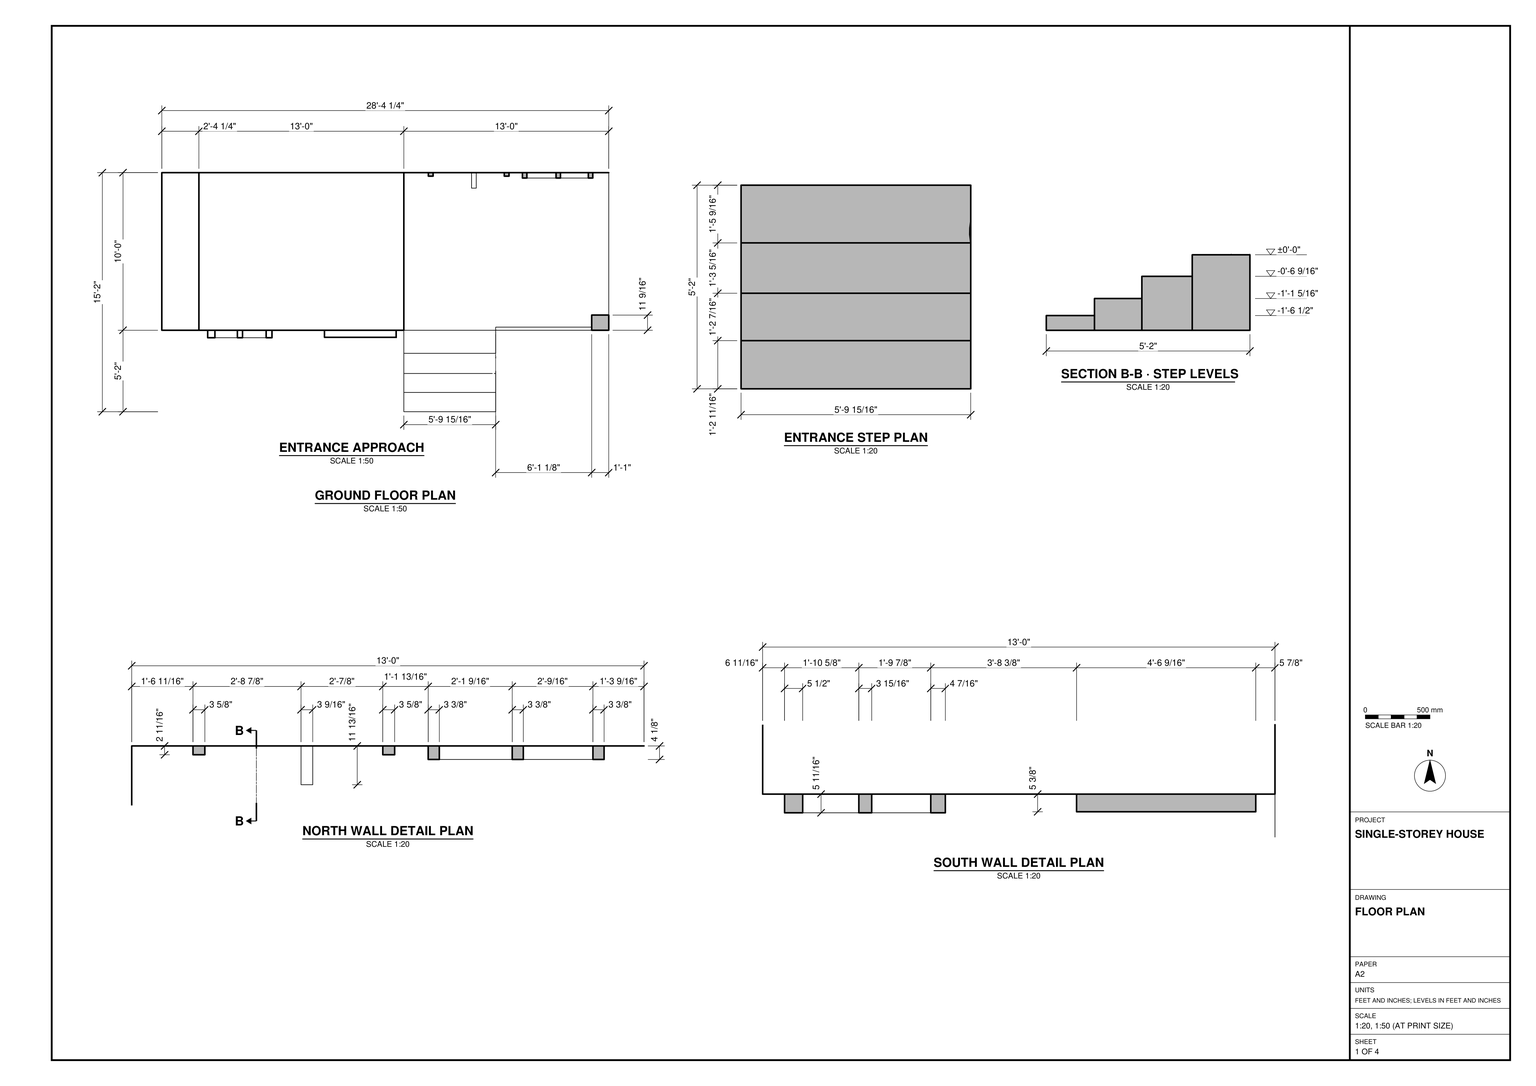
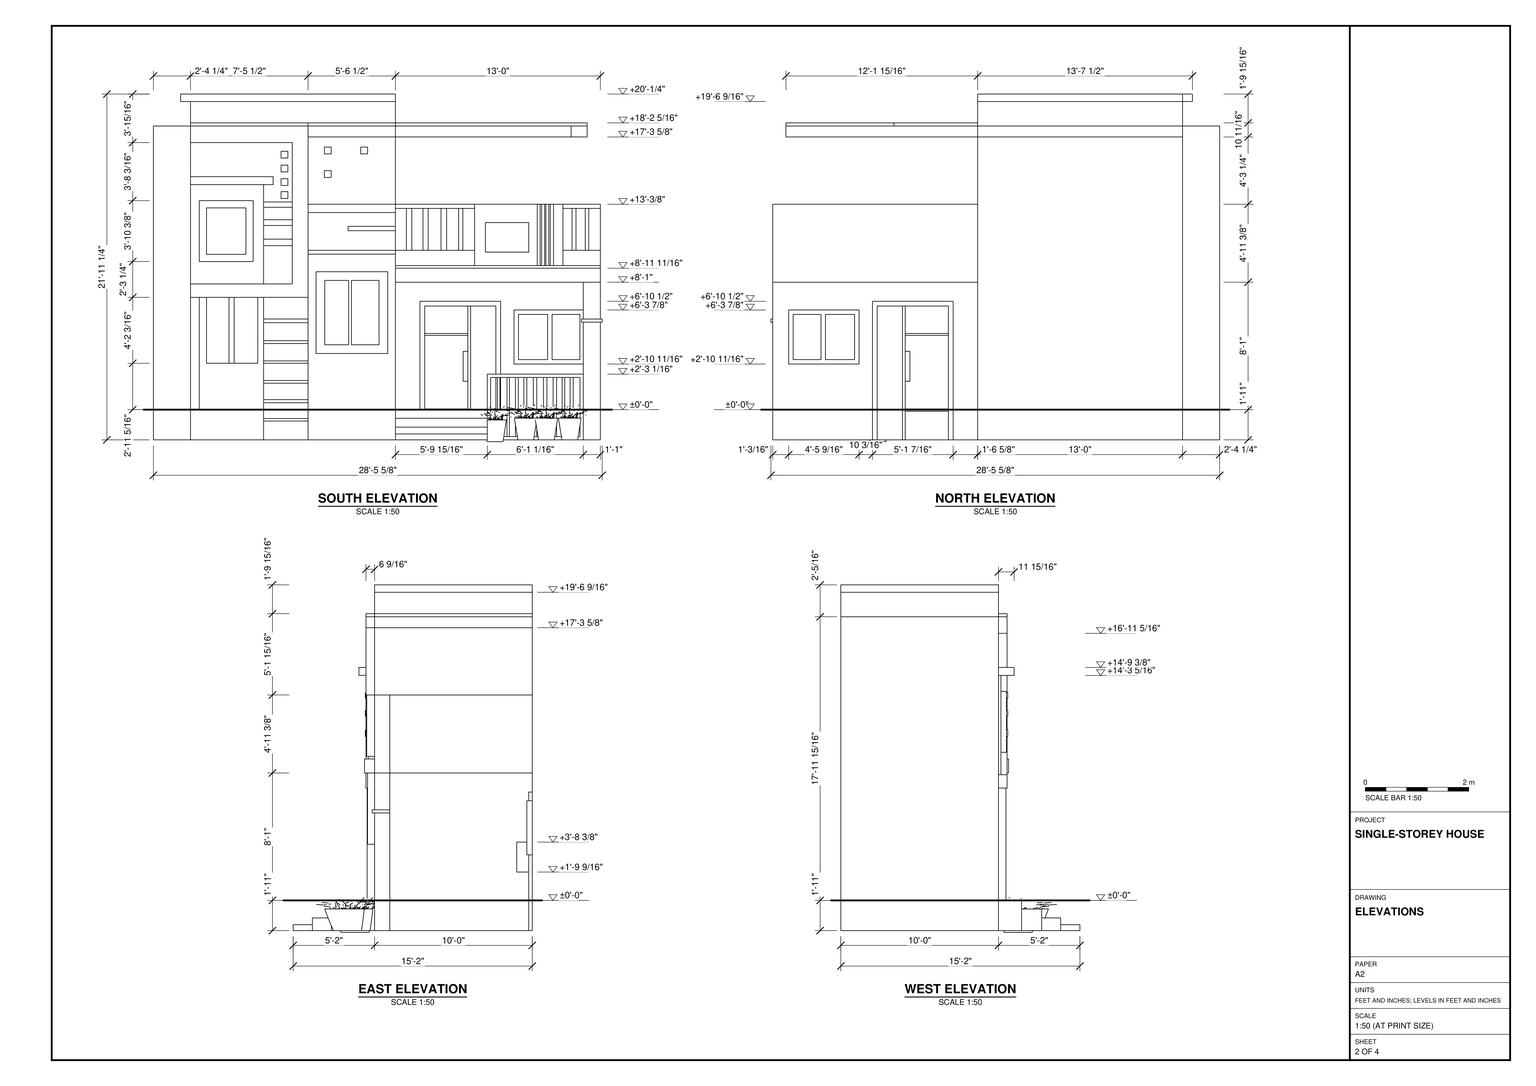
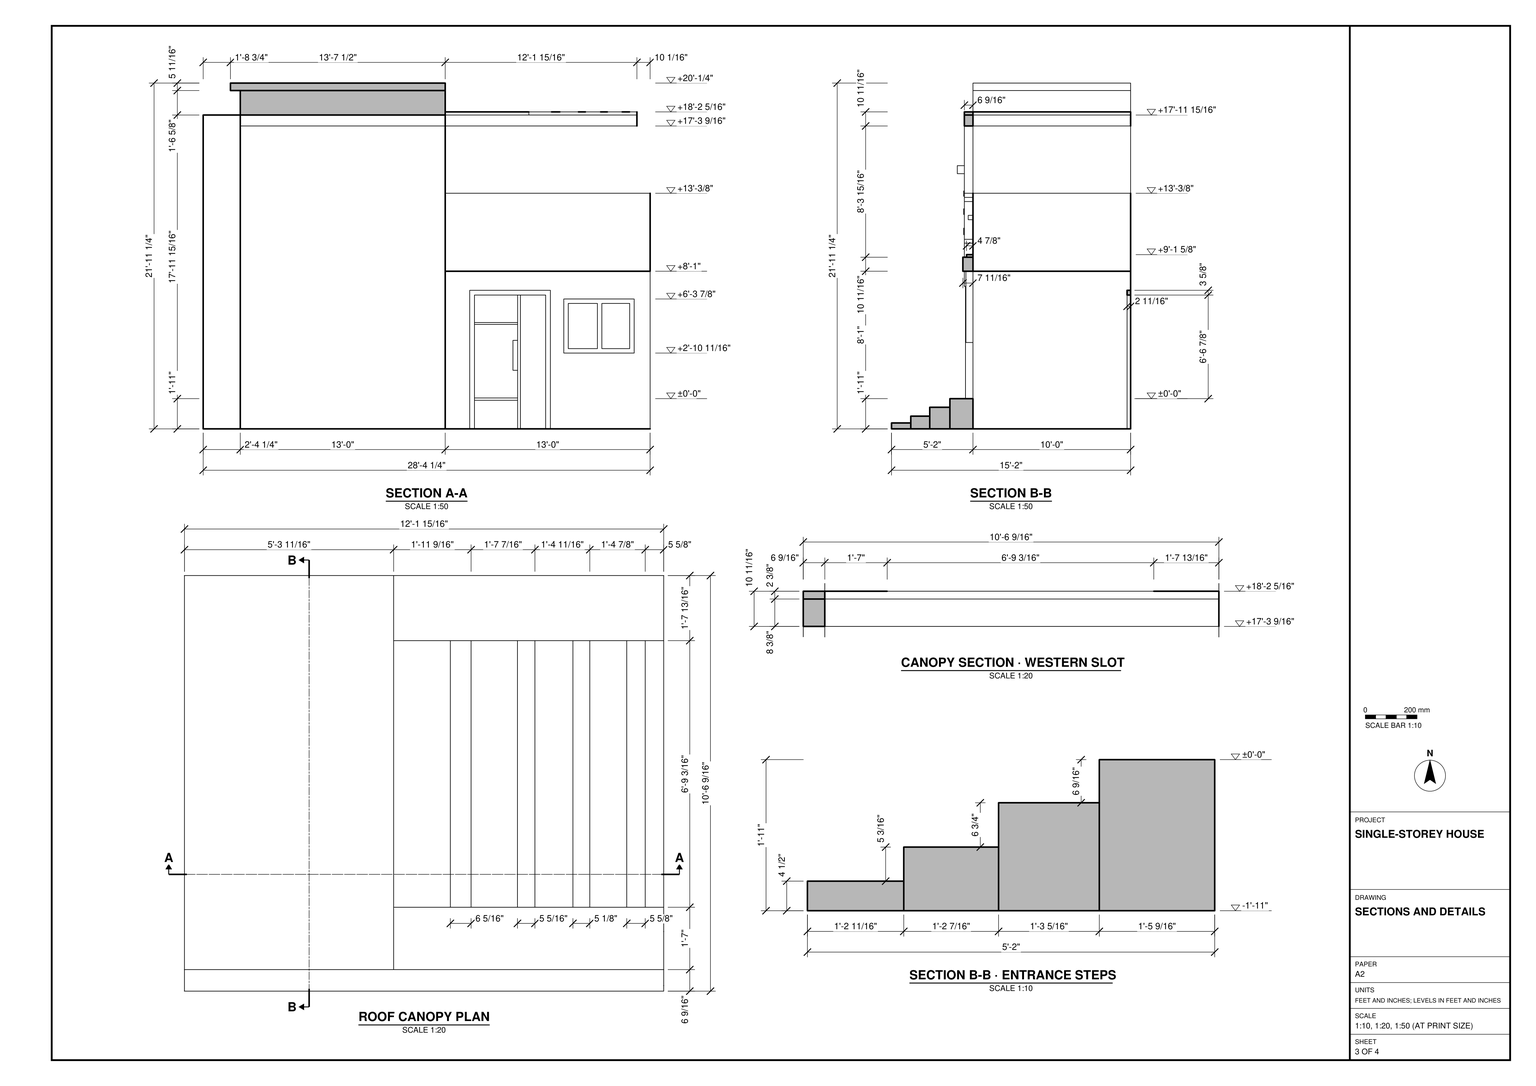
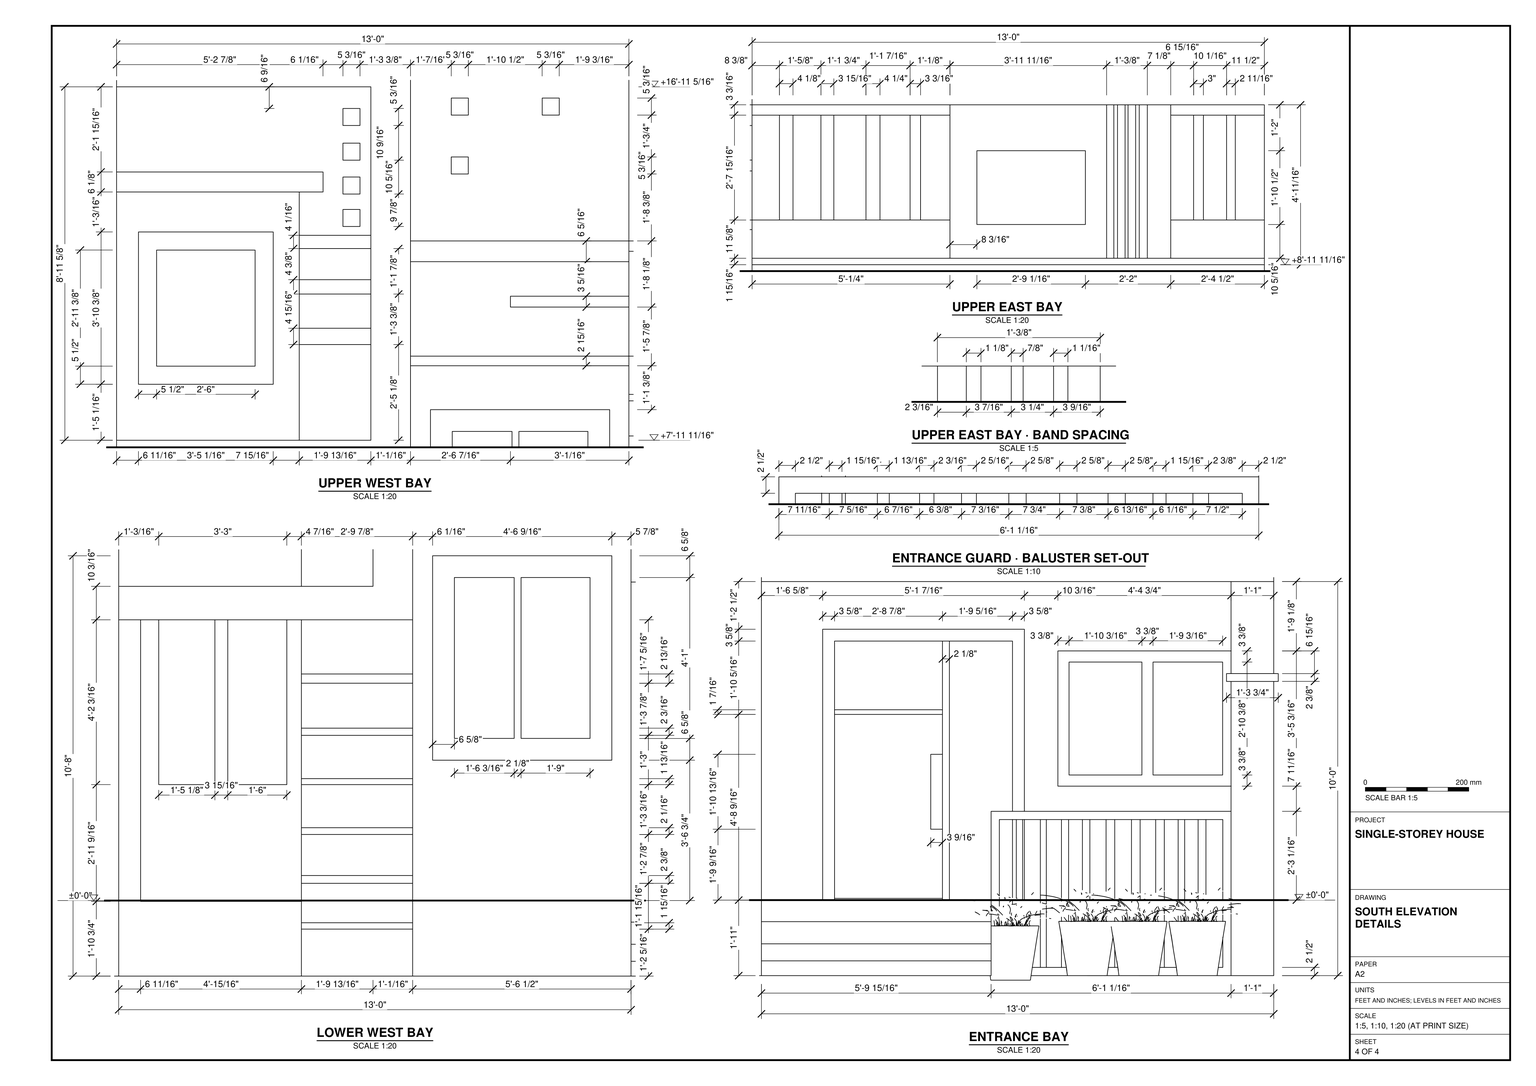
Build the single-storey house in SketchUp from task_files/diagram_01.pdf. Work in feet and inches. Set the ground floor at ±0'-0". The overall model, including projections and entrance steps, is 28'-5 5/8" wide, 15'-2" deep and 22'-5/8" high. Measure the height from the lowest base to the highest roof edge, not from the ground-floor datum.

Use the plan to lay out the 10'-0" deep house body. Place the taller capped volume to the left when viewed from the south, with the entrance in the lower bay to its right. Model the base, walls and slabs with the thicknesses, offsets and projecting edges shown in plan and section. Use the south elevation to position the framed door and window units, recessed panels, horizontal bands and vertical divisions. Follow the north elevation for the rear door and window rather than copying the front. Form the solid and slotted portions of the roof canopy from its detail plan.

Build the entrance steps to the widths, tread depths and levels shown in the step details. Include the low railing and row of planters beside the approach. Decor and loose items, including the plants, may be any suitable library components. Keep shell elements such as walls, slabs and roof, and each furniture or joinery piece, in separate groups or components; use components for repeated parts. Save one SketchUp model as output_files/single_storey_house_with_entry_steps_and_slotted_canopy.skp.

# SketchUp Ruby script. Lengths in inches.
U = 1.inch
M = Sketchup.active_model
def pt(a) = Geom::Point3d.new(a.map { |v| v * U })
def face(e, loops, mat)
  f = e.add_face(loops[0].map { |a| pt(a) })
  loops[1..].each { |l| e.add_face(l.map { |a| pt(a) }).erase! }
  f.material = f.back_material = mat if mat
  f
end
# faces: each face lists its corners as indices into pts; further lists are holes
def faces(e, pts, list, mat = nil) = list.each { |f| face(e, (f[0].is_a?(Array) ? f : [f]).map { |l| l.map { |i| pts[i] } }, mat) }
# xy, xz, yz: faces in a plane at the given z, y or x. An outline is a flat list of corners, or four numbers for a rectangle; further outlines are holes
def ring(l) = l.size == 4 ? [[l[0], l[1]], [l[2], l[1]], [l[2], l[3]], [l[0], l[3]]] : l.each_slice(2).to_a
def flat(e, list, mat, &to3) = list.each { |f| face(e, (f[0].is_a?(Array) ? f : [f]).map { |l| ring(l).map { |u, v| to3.(u, v) } }, mat) }
def xy(e, z, list, mat = nil) = flat(e, list, mat) { |x, y| [x, y, z] }
def xz(e, y, list, mat = nil) = flat(e, list, mat) { |x, z| [x, y, z] }
def yz(e, x, list, mat = nil) = flat(e, list, mat) { |y, z| [x, y, z] }
def lines(e, pts, list) = list.each { |a, b| e.add_line(pt(pts[a]), pt(pts[b])) }
# prism: a flat outline (further loops are holes) pulled along v
def prism(e, loops, v, mat = nil)
  f = face(e, loops, mat); d = Geom::Vector3d.new(v.map { |x| x * U })
  f.pushpull(f.normal.samedirection?(d) ? d.length : -d.length)
end
def box(e, o, s, mat = nil) = prism(e, [[o, [o[0] + s[0], o[1], o[2]], [o[0] + s[0], o[1] + s[1], o[2]], [o[0], o[1] + s[1], o[2]]]], [0, 0, s[2]], mat)
def at(x, y, z, deg = 0) = Geom::Transformation.translation(pt([x, y, z])) * Geom::Transformation.rotation(ORIGIN, Z_AXIS, deg.degrees)
def axes(o, x, y, z) = Geom::Transformation.new([*x, 0, *y, 0, *z, 0, *pt(o).to_a, 1])
def part(name) = M.definitions.add(name)
# library, detail: a bought-in or finely detailed component or shape, given as its bounding box
def library(name, o, s) = part(name).tap { |d| box(d.entities, o, s) }
def detail(e, o, s) = box(e.add_group.entities, o, s)
def put(e, d, t, mat = nil) = e.add_instance(d, t).tap { |i| i.material = mat if mat }
def group(e, t, mat = nil) = e.add_group.tap { |g| g.transformation = t; g.material = mat if mat }.entities
root = M.entities
M.materials.add("Material__1").color = [51, 42, 44]
M.materials.add("Material__2").color = [97, 132, 37]
M.materials.add("[0018_Brown]").color = [165, 42, 42]
M.materials.add("[0022_Maroon]").color = [128, 0, 0]
M.materials.add("[0040_Peru]").color = [205, 133, 63]
M.materials.add("[0078_DarkSlateGray]").color = [47, 79, 79]
M.materials.add("[0110_LightSlateGray]").color = [119, 136, 153]
M.materials.add("[0111_SlateGray]").color = [112, 128, 144]
M.materials.add("[0117_GhostWhite]").color = [248, 248, 255]
M.materials.add("[Brick Tumbled]").color = [135, 132, 132]
M.materials.add("[Metal Seamed]").color = [118, 119, 115]
M.materials.add("[Translucent Glass Dark Green]").color = [62, 91, 5]
M.materials["[Translucent Glass Dark Green]"].alpha = 0.5
M.materials.add("[Translucent Glass Sky Reflection]").color = [126, 138, 183]
M.materials["[Translucent Glass Sky Reflection]"].alpha = 0.52
c1 = library("\#1",[-138.85,-135.75,0],[277.7,270.97,9.64])
c2 = library("\#2",[-34.84,-73.35,-33.91],[69.68,146.26,68.31])
c3 = library("\#5",[-4127.85,-1300.75,-2324.72],[5349.84,4521.24,5423.31])
c4 = part("\#3")
put(c4.entities,c3,at(450.18,-1111.4375,0),"Material__2")
c5 = part("12")
put(c5.entities,c1,axes([-49.79,-36.9375,349.64],[0.59279,0,0],[0,0.59279,0],[0,0,0.59279]),"Material__1")
put(c5.entities,c2,axes([-39.24,-18.18,177.19],[1.20819,-2.09264,0],[0,0,2.41638],[2.09264,1.20819,0]))
put(c5.entities,c4,axes([-83.44,-46.04,442.44],[-0.03636,-0.03293,-0.01473],[-0.00083,-0.02391,0.05549],[0.02997,-0.02791,-0.01158]))
xy(root,0,[[184.25,0,254.1875,14.67],[184.25,14.67,254.1875,29.1],[184.25,29.1,254.1875,44.44],[184.25,44.44,254.1875,62.01],[0,62.01,28.25,182.01],
  [28.25,62.01,184.25,182.01],[184.25,62.01,184.25,182.01,202.91,182.01,202.91,179.32,206.52,179.32,206.52,182.01,260.71,182.01,260.71,179.32,264.32,179.32,264.32,182.01,340.25,182.01,340.25,73.59,327.25,73.59,327.25,64.39,254.1875,64.39,254.1875,62.01],[254.1875,62.01,327.25,64.39],[327.25,62.01,340.25,73.59],[202.91,179.32,206.52,182.01],
  [260.71,179.32,264.32,182.01]])
xy(root,4.5,[[184.25,0,254.1875,14.67]])
xy(root,9.6875,[[184.25,14.67,254.1875,29.1]])
xy(root,16.4375,[[184.25,29.1,254.1875,44.44]])
xy(root,22.75,[[34.92,56.32,83.875,62.01]])
xy(root,23,[[184.25,44.44,254.1875,62.01]])
xy(root,44.58,[[235.81,170.2,239.37,182.01]],"[0040_Peru]")
xy(root,50.03,[[254.1875,62.01,327.25,64.39]])
xy(root,57.7,[[274.52,177.89,328.09,182.01]])
xy(root,58.3125,[[40.4375,56.32,57.53,62.01],[57.53,56.32,61.45,62.01],[61.45,56.32,79.4375,62.01]])
xy(root,61.09,[[277.92,177.89,300.11,182.01],[303.5,177.89,324.69,182.01]])
xy(root,65.75,[[123.83,56.64,178.4,62.01]])
xy(root,67.4,[[235.81,170.2,239.37,182.01]],"[0040_Peru]")
xy(root,72.375,[[130.46,56.64,148.66,62.01],[150.76,56.64,171.77,62.01]])
xy(root,89.59,[[325.875,60.14,325.875,73.59,327.25,73.59,327.25,62.01,340.25,62.01,340.25,73.59,341.625,73.59,341.625,60.14]])
xy(root,91.98,[[325.875,60.14,341.625,60.14,341.625,73.59,340.25,73.59,340.25,62.01,327.25,62.01,327.25,73.59,325.875,73.59]])
xy(root,95.49,[[277.92,177.89,300.11,182.01],[303.5,177.89,324.69,182.01]])
xy(root,98.88,[[274.52,177.89,328.09,182.01]])
xy(root,101.875,[[206.52,179.32,260.71,182.01]])
xy(root,105.49,[[202.91,179.32,264.32,182.01]])
xy(root,108.5,[[28.25,55.45,34.92,62.01],[34.92,55.45,40.4375,56.32],[40.4375,55.45,57.53,62.01],[57.53,55.45,61.45,56.32],[61.45,55.45,79.4375,62.01],
  [79.4375,55.45,83.875,56.32],[83.875,55.45,117.76,62.01],[34.92,56.32,40.4375,62.01],[57.53,56.32,61.45,62.01],[79.4375,56.32,83.875,62.01]])
xy(root,118.6875,[[28.25,55.45,83.875,60.14],[83.875,55.45,105.68,62.01],[28.25,60.14,83.875,62.01],[28.25,62.01,83.875,66.26]])
xy(root,120,[[184.25,54.32,327.25,62.01],[327.25,54.32,340.25,62.01],[184.25,62.01,184.25,182.01,340.25,182.01,340.25,73.59,327.25,73.59,327.25,62.01],[327.25,62.01,340.25,73.59]])
xy(root,121.375,[[130.46,56.64,148.66,62.01],[150.76,56.64,171.77,62.01]])
xy(root,128,[[123.83,56.64,178.4,62.01]])
xy(root,130.6875,[[184.25,54.32,340.25,57.14],[184.25,57.14,340.25,62.01]])
xy(root,132.65,[[244.51,56.01,311.75,57.14],[184.25,57.14,244.51,62.01],[244.51,57.14,311.75,62.01],[311.75,57.14,340.25,62.01]])
xy(root,135.73,[[34.92,55.89,75.95,60.14],[34.92,60.14,75.95,62.01],[34.92,62.01,75.95,66.26]])
xy(root,141.25,[[40.4375,55.89,70.4375,62.01]])
xy(root,142.93,[[252.72,56.01,285.75,57.89]])
xy(root,147.83,[[83.875,54.95,105.68,62.01]],"[0078_DarkSlateGray]")
xy(root,152.79,[[83.875,54.95,105.68,62.01]],"[0078_DarkSlateGray]")
xy(root,159.24,[[148.1875,58.39,184.25,62.01]])
xy(root,162.55,[[148.1875,58.39,184.25,62.01]])
xy(root,163.22,[[83.875,54.95,105.68,62.01]],"[0078_DarkSlateGray]")
xy(root,165.4,[[252.72,56.01,285.75,57.89]])
xy(root,167.58,[[83.875,54.95,105.68,62.01]],"[0078_DarkSlateGray]")
xy(root,173.07,[[117.76,55.45,184.25,62.01]])
xy(root,176.6,[[40.4375,55.89,70.4375,62.01]])
xy(root,177.0625,[[83.875,54.95,105.68,62.01]],"[0078_DarkSlateGray]")
xy(root,179.38,[[117.76,55.45,184.25,62.01],[244.51,56.01,311.75,62.01]])
xy(root,181.1,[[83.875,54.95,105.68,62.01]],"[0078_DarkSlateGray]")
xy(root,182.12,[[34.92,55.89,75.95,60.14],[34.92,60.14,75.95,62.01],[34.92,62.01,75.95,66.26]])
xy(root,194.29,[[28.25,50.07,83.875,60.14],[83.875,50.07,91.125,62.01],[28.25,60.14,83.875,62.01],[28.25,62.01,83.875,66.26]])
xy(root,200.375,[[28.25,50.07,91.125,62.01]])
xy(root,226.32,[[28.25,55.45,105.68,62.01]])
xy(root,230.6,[[117.76,55.45,184.25,62.01],[184.25,55.45,330.1875,62.01]])
xy(root,238.9375,[[28.25,55.45,117.76,62.01],[117.76,55.45,184.25,62.01],[184.25,55.45,330.1875,62.01],[0,62.01,28.25,182.01],[28.25,62.01,184.25,182.01]])
xy(root,241.3125,[[28.25,55.45,117.76,62.01],[117.76,55.45,184.25,62.01],[184.25,55.45,330.1875,62.01]])
xy(root,241.3125,[[184.25,62.01,247.95,182.01],[247.95,62.01,330.1875,80.99],[265.22,80.99,271.53,162.18],[285.65,80.99,290.97,162.18],[302.54,80.99,307.68,162.18],
  [318.93,80.99,324.56,162.18],[247.95,162.18,330.1875,182.01]],"[0022_Maroon]")
xy(root,257.5625,[[20.75,62.01,28.25,182.01],[28.25,62.01,184.25,182.01]])
xy(root,263.25,[[20.75,62.01,184.25,182.01]])
xz(root,0,[[184.25,0,254.1875,4.5]])
xz(root,14.67,[[184.25,0,254.1875,4.5],[184.25,4.5,254.1875,9.6875]])
xz(root,29.1,[[184.25,0,254.1875,9.6875],[184.25,9.6875,254.1875,16.4375]])
xz(root,44.44,[[184.25,0,254.1875,16.4375],[184.25,16.4375,254.1875,23]])
xz(root,50.07,[[28.25,194.29,91.125,200.375]])
xz(root,54.32,[[184.25,120,340.25,130.6875]],"[0110_LightSlateGray]")
xz(root,54.95,[[83.875,147.83,105.68,152.79],[83.875,163.22,105.68,167.58],[83.875,177.0625,105.68,181.1]],"[0078_DarkSlateGray]")
xz(root,55.45,[[28.25,108.5,117.76,108.5,117.76,238.9375,28.25,238.9375,28.25,226.32,105.68,226.32,105.68,118.6875,28.25,118.6875],[117.76,173.07,184.25,179.38],[117.76,230.6,184.25,238.9375],[184.25,230.6,317.99,238.9375],[317.99,230.6,330.1875,238.9375],
  [28.25,238.9375,117.76,241.3125],[117.76,238.9375,184.25,241.3125],[184.25,238.9375,330.1875,241.3125]])
xz(root,55.89,[[[34.92,135.73,75.95,182.12],[40.4375,141.25,70.4375,176.6]]])
xz(root,56.01,[[292.22,132.65,294.42,179.38],[295.53,132.65,297.84,179.38],[298.74,132.65,301.0625,179.38],[302.15,132.65,304.61,179.38]])
xz(root,56.01,[[[244.51,132.65,292.22,179.38],[252.72,142.93,285.75,165.4]],[294.42,132.65,295.53,179.38],[297.84,132.65,298.74,179.38],[301.0625,132.65,302.15,179.38],[304.61,132.65,311.75,179.38]],"[0111_SlateGray]")
xz(root,56.32,[[34.92,22.75,83.875,22.75,83.875,108.5,79.4375,108.5,79.4375,58.3125,40.4375,58.3125,40.4375,108.5,34.92,108.5],[57.53,58.3125,61.45,108.5]])
xz(root,56.64,[[[123.83,65.75,178.4,128],[150.76,72.375,171.77,121.375],[130.46,72.375,148.66,121.375]]])
xz(root,57.14,[[184.25,130.6875,340.25,132.65]])
xz(root,57.89,[[252.72,142.93,285.75,165.4]])
xz(root,58.39,[[148.1875,159.24,184.25,162.55]])
xz(root,60.14,[[325.875,89.59,341.625,91.98]])
xz(root,60.14,[[[28.25,118.6875,83.875,194.29],[34.92,135.73,75.95,182.12]]],"[0110_LightSlateGray]")
xz(root,62.01,[[83.875,0,117.76,14.31],[184.25,0,254.1875,23],[83.875,16.24,117.76,28.25],[34.92,22.75,34.92,108.5,40.4375,108.5,40.4375,58.3125,79.4375,58.3125,79.4375,108.5,83.875,108.5,83.875,22.75],[83.875,30.625,117.76,43.125],
  [83.875,45.1875,117.76,58.3125],[57.53,58.3125,61.45,108.5],[83.875,60.125,117.76,73.3125],[[123.83,65.75,178.4,128],[150.76,72.375,171.77,121.375],[130.46,72.375,148.66,121.375]],[83.875,75.5,117.76,89.1875],
  [327.25,89.59,340.25,91.98],[327.25,91.98,340.25,120],[83.875,92,117.76,108.5],[28.25,108.5,28.25,118.6875,105.68,118.6875,105.68,226.32,28.25,226.32,28.25,238.9375,117.76,238.9375,117.76,108.5],[[28.25,118.6875,83.875,194.29],[34.92,135.73,75.95,182.12]],
  [83.875,118.6875,105.68,147.83],[184.25,120,340.25,130.6875],[184.25,130.6875,340.25,132.65],[184.25,132.65,244.51,144.3],[244.51,132.65,311.75,179.38],
  [311.75,132.65,340.25,144.3],[[34.92,135.73,75.95,182.12],[40.4375,141.25,70.4375,176.6]],[117.76,141.375,184.25,144.3],[83.875,147.83,105.68,152.79],[83.875,152.79,105.68,163.22],
  [148.1875,159.24,184.25,162.55],[83.875,163.22,105.68,167.58],[83.875,167.58,105.68,177.0625],[117.76,173.07,184.25,179.38],[83.875,177.0625,105.68,181.1],
  [[117.76,179.38,184.25,230.6],[130.17,217.7,135.36,222.89],[157.86,217.7,163.05,222.89],[130.16,199.77,135.34,204.96]],[[83.875,181.1,105.68,181.1,105.68,226.32,28.25,226.32,28.25,200.375,91.125,200.375,91.125,194.29,83.875,194.29],[97.18,214.54,102.37,219.72],[97.18,203.97,102.37,209.16],[97.18,193.66,102.37,198.85],[97.18,183.79,102.37,188.97]],[28.25,194.29,91.125,200.375],[117.76,230.6,184.25,238.9375],[28.25,238.9375,117.76,241.3125],
  [117.76,238.9375,184.25,241.3125],[20.75,257.5625,184.25,263.25]])
xz(root,62.01,[[184.25,230.6,330.1875,238.9375],[184.25,238.9375,330.1875,241.3125]],"[0022_Maroon]")
xz(root,62.01,[[28.25,0,83.875,0,83.875,22.75,34.92,22.75,34.92,108.5,28.25,108.5],[327.25,0,340.25,89.59],[83.875,14.31,117.76,16.24],[83.875,28.25,117.76,30.625],[83.875,43.125,117.76,45.1875],
  [83.875,58.3125,117.76,60.125],[83.875,73.3125,117.76,75.5],[83.875,89.1875,117.76,92],[97.18,183.79,102.37,188.97],[97.18,193.66,102.37,198.85],
  [130.16,199.77,135.34,204.96],[97.18,203.97,102.37,209.16],[97.18,214.54,102.37,219.72],[130.17,217.7,135.36,222.89],[157.86,217.7,163.05,222.89],
  [28.25,241.3125,184.25,257.5625]],"[0110_LightSlateGray]")
xz(root,62.01,[[0,0,28.25,238.9375],[[117.76,0,184.25,141.375],[123.83,65.75,178.4,128]],[117.76,144.3,184.25,144.3,184.25,159.24,148.1875,159.24,148.1875,162.55,184.25,162.55,184.25,173.07,117.76,173.07]],"[0111_SlateGray]")
xz(root,62.01,[[[254.1875,0,327.25,50.03],[256.7,2.51,324.74,47.52]],[261.86,2.51,263.8,47.52],[269.18,2.51,271,47.52],[275.61,2.51,277.8,47.52],[281.99,2.51,284.26,47.52],
  [289.2,2.51,291.84,47.52],[296.94,2.51,299.57,47.52],[304.3,2.51,306.93,47.52],[311.14,2.51,313.14,47.52],[317.23,2.51,319.61,47.52],
  [192.6,144.3,196.72,176.22],[205.22,144.3,209.15,176.22],[218.94,144.3,223.21,176.22],[232.375,144.3,235.56,176.22],[318.7,144.3,321.69,176.22],
  [328.74,144.3,331.4,176.22],[184.25,176.22,244.51,179.38],[311.75,176.22,340.25,179.38]],"[Metal Seamed]")
xz(root,62.01,[[40.4375,58.3125,57.53,108.5],[61.45,58.3125,79.4375,108.5],[130.46,72.375,148.66,121.375],[150.76,72.375,171.77,121.375]],"[Translucent Glass Dark Green]")
xz(root,62.01,[[40.4375,141.25,70.4375,176.6]],"[Translucent Glass Sky Reflection]")
xz(root,66.26,[[[28.25,118.6875,83.875,194.29],[34.92,135.73,75.95,182.12]]])
xz(root,73.59,[[325.875,89.59,327.25,91.98],[340.25,89.59,341.625,91.98]])
xz(root,73.59,[[327.25,0,340.25,120]],"[0110_LightSlateGray]")
xz(root,170.2,[[235.81,44.58,239.37,67.4]],"[0040_Peru]")
xz(root,177.89,[[[274.52,57.7,328.09,98.88],[277.92,61.09,300.11,95.49],[303.5,61.09,324.69,95.49]]])
xz(root,179.32,[[202.91,0,206.52,0,206.52,101.875,260.71,101.875,260.71,0,264.32,0,264.32,105.49,202.91,105.49]],"[0022_Maroon]")
xz(root,182.01,[[0,0,28.25,238.9375],[28.25,0,184.25,230.6],[202.91,0,202.91,105.49,264.32,105.49,264.32,0,260.71,0,260.71,101.875,206.52,101.875,206.52,0],[[274.52,57.7,328.09,98.88],[277.92,61.09,300.11,95.49],[303.5,61.09,324.69,95.49]],[184.25,120,340.25,179.38],
  [28.25,230.6,184.25,238.9375],[28.25,238.9375,184.25,257.5625],[20.75,257.5625,28.25,263.25],[28.25,257.5625,184.25,263.25]])
xz(root,182.01,[[235.81,44.58,239.37,67.4]],"[0018_Brown]")
xz(root,182.01,[[239.37,0,241.49,101.875],[206.52,21.75,239.37,23.52],[206.52,23.52,206.52,79.54,239.37,79.54,239.37,67.4,235.81,67.4,235.81,44.58,239.37,44.58,239.37,23.52],[206.52,79.54,239.37,80.97],[184.25,230.6,330.1875,238.9375],
  [184.25,238.9375,247.95,241.3125],[247.95,238.9375,330.1875,241.3125]],"[0022_Maroon]")
xz(root,182.01,[[206.52,0,239.37,21.75],[206.52,80.97,239.37,101.875]],"[0040_Peru]")
xz(root,182.01,[[241.49,0,260.71,101.875]],"[0117_GhostWhite]")
xz(root,182.01,[[[184.25,0,184.25,120,340.25,120,340.25,0,264.32,0,264.32,105.49,202.91,105.49,202.91,0],[274.52,57.7,328.09,98.88]]],"[Brick Tumbled]")
xz(root,182.01,[[277.92,61.09,300.11,95.49],[303.5,61.09,324.69,95.49]],"[Translucent Glass Sky Reflection]")
yz(root,0,[[62.01,0,182.01,238.9375]])
yz(root,20.75,[[62.01,257.5625,182.01,263.25]])
yz(root,28.25,[[62.01,0,182.01,0,182.01,238.9375,62.01,238.9375,62.01,194.29,66.26,194.29,66.26,118.6875,62.01,118.6875],[55.45,108.5,62.01,118.6875],[60.14,118.6875,62.01,194.29],[62.01,118.6875,66.26,194.29],[50.07,194.29,62.01,200.375],
  [55.45,226.32,62.01,238.9375],[55.45,238.9375,62.01,241.3125],[62.01,238.9375,182.01,257.5625]])
yz(root,34.92,[[56.32,22.75,62.01,108.5],[55.89,135.73,60.14,182.12],[60.14,135.73,62.01,182.12],[62.01,135.73,66.26,182.12]])
yz(root,40.4375,[[56.32,58.3125,62.01,108.5],[55.89,141.25,62.01,176.6]])
yz(root,57.53,[[56.32,58.3125,62.01,108.5]])
yz(root,61.45,[[56.32,58.3125,62.01,108.5]])
yz(root,70.4375,[[55.89,141.25,62.01,176.6]])
yz(root,75.95,[[55.89,135.73,60.14,182.12],[60.14,135.73,62.01,182.12],[62.01,135.73,66.26,182.12]])
yz(root,79.4375,[[56.32,58.3125,62.01,108.5]])
yz(root,83.875,[[56.32,22.75,62.01,108.5],[60.14,118.6875,62.01,147.83],[62.01,118.6875,66.26,147.83],[60.14,147.83,62.01,152.79],[62.01,147.83,66.26,152.79],
  [60.14,152.79,62.01,163.22],[62.01,152.79,66.26,163.22],[60.14,163.22,62.01,167.58],[62.01,163.22,66.26,167.58],[60.14,167.58,62.01,177.0625],
  [62.01,167.58,66.26,177.0625],[60.14,177.0625,62.01,181.1],[62.01,177.0625,66.26,181.1],[60.14,181.1,62.01,194.29],[62.01,181.1,66.26,194.29]])
yz(root,83.875,[[54.95,147.83,60.14,152.79],[54.95,163.22,60.14,167.58],[54.95,177.0625,60.14,181.1]],"[0078_DarkSlateGray]")
yz(root,91.125,[[50.07,194.29,62.01,200.375]])
yz(root,105.68,[[55.45,118.6875,62.01,147.83],[54.95,147.83,55.45,152.79],[55.45,147.83,62.01,152.79],[55.45,152.79,62.01,163.22],[54.95,163.22,55.45,167.58],
  [55.45,163.22,62.01,167.58],[55.45,167.58,62.01,177.0625],[54.95,177.0625,55.45,181.1],[55.45,177.0625,62.01,181.1],[55.45,181.1,62.01,226.32]])
yz(root,117.76,[[55.45,108.5,62.01,141.375],[55.45,141.375,62.01,144.3],[55.45,144.3,62.01,173.07],[55.45,173.07,62.01,179.38],[55.45,179.38,62.01,230.6],
  [55.45,230.6,62.01,238.9375],[55.45,238.9375,62.01,241.3125]])
yz(root,123.83,[[56.64,65.75,62.01,128]])
yz(root,130.46,[[56.64,72.375,62.01,121.375]])
yz(root,148.1875,[[58.39,159.24,62.01,162.55]])
yz(root,148.66,[[56.64,72.375,62.01,121.375]])
yz(root,150.76,[[56.64,72.375,62.01,121.375]])
yz(root,171.77,[[56.64,72.375,62.01,121.375]])
yz(root,178.4,[[56.64,65.75,62.01,128]])
yz(root,184.25,[[0,0,14.67,4.5],[14.67,0,29.1,9.6875],[29.1,0,44.44,16.4375],[44.44,0,62.01,23],[62.01,0,182.01,120],
  [54.32,120,62.01,130.6875],[62.01,120,182.01,179.38],[57.14,130.6875,62.01,132.65],[58.39,159.24,62.01,162.55],[55.45,173.07,62.01,176.22],
  [55.45,176.22,62.01,179.38],[62.01,179.38,182.01,230.6],[55.45,230.6,62.01,238.9375],[55.45,238.9375,62.01,241.3125],[62.01,241.3125,182.01,257.5625],
  [62.01,257.5625,182.01,263.25]])
yz(root,184.25,[[62.01,230.6,182.01,238.9375],[62.01,238.9375,182.01,241.3125]],"[0022_Maroon]")
yz(root,202.91,[[179.32,0,182.01,105.49]])
yz(root,206.52,[[179.32,0,182.01,101.875]])
yz(root,235.81,[[170.2,44.58,182.01,67.4]],"[0040_Peru]")
yz(root,239.37,[[170.2,44.58,182.01,67.4]],"[0040_Peru]")
yz(root,244.51,[[56.01,132.65,62.01,179.38]])
yz(root,252.72,[[56.01,142.93,57.89,165.4]])
yz(root,254.1875,[[0,0,14.67,4.5],[14.67,0,29.1,9.6875],[29.1,0,44.44,16.4375],[44.44,0,62.01,23],[62.01,0,64.39,50.03]])
yz(root,260.71,[[179.32,0,182.01,101.875]])
yz(root,264.32,[[179.32,0,182.01,105.49]])
yz(root,274.52,[[177.89,57.7,182.01,98.88]])
yz(root,277.92,[[177.89,61.09,182.01,95.49]])
yz(root,285.75,[[56.01,142.93,57.89,165.4]])
yz(root,300.11,[[177.89,61.09,182.01,95.49]])
yz(root,303.5,[[177.89,61.09,182.01,95.49]])
yz(root,311.75,[[56.01,132.65,62.01,179.38]])
yz(root,324.69,[[177.89,61.09,182.01,95.49]])
yz(root,325.875,[[60.14,89.59,73.59,91.98]])
yz(root,327.25,[[62.01,0,64.39,50.03],[62.01,89.59,73.59,91.98],[62.01,91.98,73.59,120]])
yz(root,327.25,[[64.39,0,64.39,50.03,62.01,50.03,62.01,89.59,73.59,89.59,73.59,0]],"[0110_LightSlateGray]")
yz(root,328.09,[[177.89,57.7,182.01,98.88]])
yz(root,330.1875,[[55.45,230.6,62.01,238.9375],[55.45,238.9375,62.01,241.3125]])
yz(root,330.1875,[[62.01,230.6,182.01,238.9375],[62.01,238.9375,182.01,241.3125]],"[0022_Maroon]")
yz(root,340.25,[[62.01,89.59,73.59,91.98],[62.01,91.98,73.59,120],[54.32,120,62.01,130.6875],[62.01,120,73.59,179.38],[73.59,120,182.01,179.38],
  [57.14,130.6875,62.01,132.65]])
yz(root,340.25,[[62.01,0,73.59,89.59]],"[0110_LightSlateGray]")
yz(root,341.625,[[60.14,89.59,73.59,91.98]])
put(root,c5,axes([288.53,52.22,0],[0.1027,0,0],[0,0.18206,0],[0,0,0.0468]))
put(root,c5,axes([265.19,51.56,-1.38],[0.1027,0,0],[0,0.18206,0],[0,0,0.0468]))
put(root,c5,axes([304.22,52.22,0],[0.1027,0,0],[0,0.18206,0],[0,0,0.0468]))
put(root,c5,axes([304.22,45.72,0],[0.1027,0,0],[0,0.18206,0],[0,0,0.0468]))
put(root,c5,axes([322.03,45.72,0],[0.1027,0,0],[0,0.18206,0],[0,0,0.0468]))
